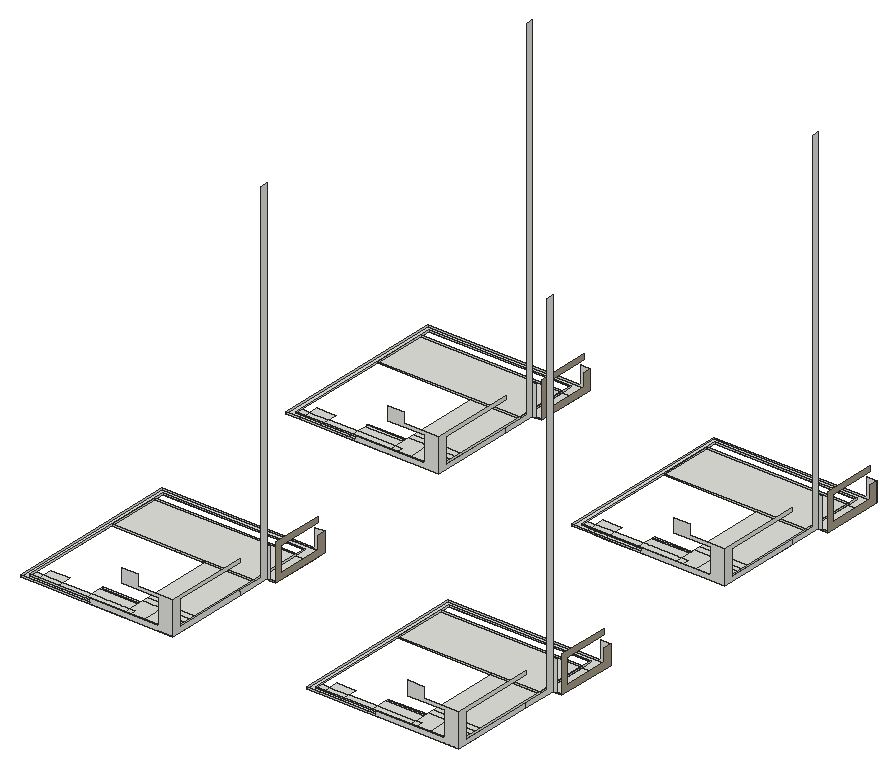
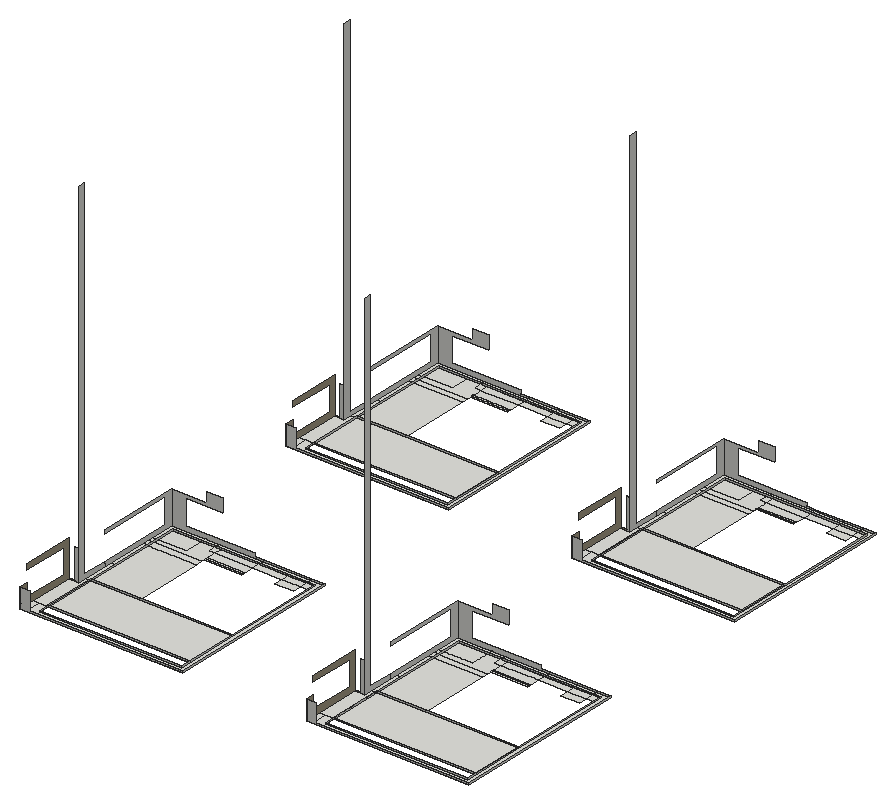
# SketchUp Ruby script. Lengths in inches.
U = 1.inch
M = Sketchup.active_model
def pt(a) = Geom::Point3d.new(a.map { |v| v * U })
def face(e, loops, mat)
  f = e.add_face(loops[0].map { |a| pt(a) })
  loops[1..].each { |l| e.add_face(l.map { |a| pt(a) }).erase! }
  f.material = f.back_material = mat if mat
  f
end
# faces: each face lists its corners as indices into pts; further lists are holes
def faces(e, pts, list, mat = nil) = list.each { |f| face(e, (f[0].is_a?(Array) ? f : [f]).map { |l| l.map { |i| pts[i] } }, mat) }
# xy, xz, yz: faces in a plane at the given z, y or x. An outline is a flat list of corners, or four numbers for a rectangle; further outlines are holes
def ring(l) = l.size == 4 ? [[l[0], l[1]], [l[2], l[1]], [l[2], l[3]], [l[0], l[3]]] : l.each_slice(2).to_a
def flat(e, list, mat, &to3) = list.each { |f| face(e, (f[0].is_a?(Array) ? f : [f]).map { |l| ring(l).map { |u, v| to3.(u, v) } }, mat) }
def xy(e, z, list, mat = nil) = flat(e, list, mat) { |x, y| [x, y, z] }
def xz(e, y, list, mat = nil) = flat(e, list, mat) { |x, z| [x, y, z] }
def yz(e, x, list, mat = nil) = flat(e, list, mat) { |y, z| [x, y, z] }
def lines(e, pts, list) = list.each { |a, b| e.add_line(pt(pts[a]), pt(pts[b])) }
# prism: a flat outline (further loops are holes) pulled along v
def prism(e, loops, v, mat = nil)
  f = face(e, loops, mat); d = Geom::Vector3d.new(v.map { |x| x * U })
  f.pushpull(f.normal.samedirection?(d) ? d.length : -d.length)
end
def box(e, o, s, mat = nil) = prism(e, [[o, [o[0] + s[0], o[1], o[2]], [o[0] + s[0], o[1] + s[1], o[2]], [o[0], o[1] + s[1], o[2]]]], [0, 0, s[2]], mat)
def at(x, y, z, deg = 0) = Geom::Transformation.translation(pt([x, y, z])) * Geom::Transformation.rotation(ORIGIN, Z_AXIS, deg.degrees)
def axes(o, x, y, z) = Geom::Transformation.new([*x, 0, *y, 0, *z, 0, *pt(o).to_a, 1])
def part(name) = M.definitions.add(name)
# library, detail: a bought-in or finely detailed component or shape, given as its bounding box
def library(name, o, s) = part(name).tap { |d| box(d.entities, o, s) }
def detail(e, o, s) = box(e.add_group.entities, o, s)
def put(e, d, t, mat = nil) = e.add_instance(d, t).tap { |i| i.material = mat if mat }
def group(e, t, mat = nil) = e.add_group.tap { |g| g.transformation = t; g.material = mat if mat }.entities
root = M.entities
M.materials.add("[Concrete Tile]").color = [165, 155, 133]
xy(root,252,[[262.875,1799.9375,262.875,2554.375,927.75,2554.375,927.75,2483.21,890.875,2483.21,890.875,2531.375,285.875,2531.375,285.875,1822.9375,319.53,1822.9375,319.53,1799.9375],[319.53,1799.9375,399.88,1822.9375],[399.88,1799.9375,523.04,1822.9375],[523.04,1799.9375,709.87,1822.9375],[709.87,1799.9375,767.19,1822.9375],
  [767.19,1799.9375,767.19,1822.9375,890.875,1822.9375,890.875,1902.66,913.875,1902.66,913.875,1799.9375],[1481.0625,1799.9375,1481.0625,2554.375,2145.9375,2554.375,2145.9375,2483.21,2109.0625,2483.21,2109.0625,2531.375,1504.0625,2531.375,1504.0625,1822.9375,1537.72,1822.9375,1537.72,1799.9375],[1537.72,1799.9375,1618.07,1822.9375],[1618.07,1799.9375,1741.23,1822.9375],[1741.23,1799.9375,1928.05,1822.9375],
  [1928.05,1799.9375,1985.38,1822.9375],[1985.38,1799.9375,1985.38,1822.9375,2109.0625,1822.9375,2109.0625,1902.66,2132.0625,1902.66,2132.0625,1799.9375],[285.875,1822.9375,319.53,1855.75],[319.53,1822.9375,399.88,1855.75],[399.88,1822.9375,523.04,1855.75],
  [523.04,1822.9375,683.6875,1855.75],[683.6875,1822.9375,709.87,1855.75],[709.87,1822.9375,767.19,1822.9375,767.19,1902.66,890.875,1902.66,890.875,1926.07,683.6875,1926.07,683.6875,1855.75,709.87,1855.75],[767.19,1822.9375,890.875,1902.66],[1504.0625,1822.9375,1537.72,1855.75],
  [1537.72,1822.9375,1618.07,1855.75],[1618.07,1822.9375,1741.23,1855.75],[1741.23,1822.9375,1901.875,1855.75],[1901.875,1822.9375,1928.05,1855.75],[1928.05,1822.9375,1985.38,1822.9375,1985.38,1902.66,2109.0625,1902.66,2109.0625,1926.07,1901.875,1926.07,1901.875,1855.75,1928.05,1855.75],
  [1985.38,1822.9375,2109.0625,1902.66],[319.53,1855.75,399.88,1893.25],[523.04,1855.75,683.6875,1897.5625],[1537.72,1855.75,1618.07,1893.25],[1741.23,1855.75,1901.875,1897.5625],
  [523.04,1897.5625,683.6875,1906.6875],[1741.23,1897.5625,1901.875,1906.6875],[890.875,1902.66,894.3125,1926.07],[894.3125,1902.66,913.875,1926.07],[2109.0625,1902.66,2112.5,1926.07],
  [2112.5,1902.66,2132.0625,1926.07],[523.04,1906.6875,683.6875,1913.4375],[1741.23,1906.6875,1901.875,1913.4375],[683.6875,1926.07,890.875,1953.7],[890.875,1926.07,894.3125,1953.7],
  [894.3125,1926.07,913.875,1953.7],[1901.875,1926.07,2109.0625,1953.7],[2109.0625,1926.07,2112.5,1953.7],[2112.5,1926.07,2132.0625,1953.7],[683.6875,1953.7,890.875,2258.18],
  [890.875,1953.7,890.875,2258.18,913.875,2258.18,913.875,2124.51,894.3125,2124.51,894.3125,1953.7],[894.3125,1953.7,913.875,2124.51],[1901.875,1953.7,2109.0625,2258.18],[2109.0625,1953.7,2109.0625,2258.18,2132.0625,2258.18,2132.0625,2124.51,2112.5,2124.51,2112.5,1953.7],[2112.5,1953.7,2132.0625,2124.51],
  [285.875,2258.18,890.875,2486.82],[890.875,2258.18,890.875,2483.21,954.6875,2483.21,954.6875,2295.875,913.875,2295.875,913.875,2258.18],[1504.0625,2258.18,2109.0625,2486.82],[2109.0625,2258.18,2109.0625,2483.21,2172.875,2483.21,2172.875,2295.875,2132.0625,2295.875,2132.0625,2258.18],[927.75,2483.21,954.6875,2554.375],
  [2145.9375,2483.21,2172.875,2554.375],[262.875,3214.625,262.875,3969.0625,927.75,3969.0625,927.75,3897.9,890.875,3897.9,890.875,3946.0625,285.875,3946.0625,285.875,3237.625,319.53,3237.625,319.53,3214.625],[319.53,3214.625,399.88,3237.625],[399.88,3214.625,523.04,3237.625],[523.04,3214.625,709.87,3237.625],
  [709.87,3214.625,767.19,3237.625],[767.19,3214.625,767.19,3237.625,890.875,3237.625,890.875,3317.34,913.875,3317.34,913.875,3214.625],[1481.0625,3214.625,1481.0625,3969.0625,2145.9375,3969.0625,2145.9375,3897.9,2109.0625,3897.9,2109.0625,3946.0625,1504.0625,3946.0625,1504.0625,3237.625,1537.72,3237.625,1537.72,3214.625],[1537.72,3214.625,1618.07,3237.625],[1618.07,3214.625,1741.23,3237.625],
  [1741.23,3214.625,1928.05,3237.625],[1928.05,3214.625,1985.38,3237.625],[1985.38,3214.625,1985.38,3237.625,2109.0625,3237.625,2109.0625,3317.34,2132.0625,3317.34,2132.0625,3214.625],[285.875,3237.625,319.53,3270.4375],[319.53,3237.625,399.88,3270.4375],
  [399.88,3237.625,523.04,3270.4375],[523.04,3237.625,683.6875,3270.4375],[683.6875,3237.625,709.87,3270.4375],[709.87,3237.625,767.19,3237.625,767.19,3317.34,890.875,3317.34,890.875,3340.76,683.6875,3340.76,683.6875,3270.4375,709.87,3270.4375],[767.19,3237.625,890.875,3317.34],
  [1504.0625,3237.625,1537.72,3270.4375],[1537.72,3237.625,1618.07,3270.4375],[1618.07,3237.625,1741.23,3270.4375],[1741.23,3237.625,1901.875,3270.4375],[1901.875,3237.625,1928.05,3270.4375],
  [1928.05,3237.625,1985.38,3237.625,1985.38,3317.34,2109.0625,3317.34,2109.0625,3340.76,1901.875,3340.76,1901.875,3270.4375,1928.05,3270.4375],[1985.38,3237.625,2109.0625,3317.34],[319.53,3270.4375,399.88,3307.9375],[523.04,3270.4375,683.6875,3312.25],[1537.72,3270.4375,1618.07,3307.9375],
  [1741.23,3270.4375,1901.875,3312.25],[523.04,3312.25,683.6875,3321.375],[1741.23,3312.25,1901.875,3321.375],[890.875,3317.34,894.3125,3340.76],[894.3125,3317.34,913.875,3340.76],
  [2109.0625,3317.34,2112.5,3340.76],[2112.5,3317.34,2132.0625,3340.76],[523.04,3321.375,683.6875,3328.125],[1741.23,3321.375,1901.875,3328.125],[683.6875,3340.76,890.875,3368.39],
  [890.875,3340.76,894.3125,3368.39],[894.3125,3340.76,913.875,3368.39],[1901.875,3340.76,2109.0625,3368.39],[2109.0625,3340.76,2112.5,3368.39],[2112.5,3340.76,2132.0625,3368.39],
  [683.6875,3368.39,890.875,3672.87],[890.875,3368.39,890.875,3672.87,913.875,3672.87,913.875,3539.2,894.3125,3539.2,894.3125,3368.39],[894.3125,3368.39,913.875,3539.2],[1901.875,3368.39,2109.0625,3672.87],[2109.0625,3368.39,2109.0625,3672.87,2132.0625,3672.87,2132.0625,3539.2,2112.5,3539.2,2112.5,3368.39],
  [2112.5,3368.39,2132.0625,3539.2],[285.875,3672.87,890.875,3901.51],[890.875,3672.87,890.875,3897.9,954.6875,3897.9,954.6875,3710.5625,913.875,3710.5625,913.875,3672.87],[1504.0625,3672.87,2109.0625,3901.51],[2109.0625,3672.87,2109.0625,3897.9,2172.875,3897.9,2172.875,3710.5625,2132.0625,3710.5625,2132.0625,3672.87],
  [927.75,3897.9,954.6875,3969.0625],[2145.9375,3897.9,2172.875,3969.0625]])
xz(root,1799.9375,[[262.875,252,319.53,258],[319.53,252,523.04,258],[523.04,252,557.4,258],[557.4,252,913.875,252,913.875,391.25,762.28,391.25,762.28,435.5,695.43,435.5,695.43,378,852.75,378,852.75,272.125,557.88,272.125,557.88,258,557.4,258],[1481.0625,252,1537.72,258],
  [1537.72,252,1741.23,258],[1741.23,252,1775.59,258],[1775.59,252,2132.0625,252,2132.0625,391.25,1980.47,391.25,1980.47,435.5,1913.62,435.5,1913.62,378,2070.9375,378,2070.9375,272.125,1776.07,272.125,1776.07,258,1775.59,258]])
xz(root,1822.9375,[[285.875,252,890.875,258],[1504.0625,252,2109.0625,258]])
xz(root,2258.18,[[285.875,252,683.6875,257.875],[683.6875,252,890.875,257.875],[1504.0625,252,1901.875,257.875],[1901.875,252,2109.0625,257.875]])
xz(root,2295.875,[[913.875,252,930.75,384],[2132.0625,252,2148.9375,384]])
xz(root,2295.875,[[930.75,252,954.6875,258],[2148.9375,252,2172.875,258]],"[Concrete Tile]")
xz(root,2486.82,[[285.875,252,890.875,257.875],[1504.0625,252,2109.0625,257.875]])
xz(root,2531.375,[[285.875,252,890.875,258],[1504.0625,252,2109.0625,258]])
xz(root,2554.375,[[262.875,252,262.875,258,913.875,258,913.875,336.0625,954.6875,336.0625,954.6875,252],[1481.0625,252,1481.0625,258,2132.0625,258,2132.0625,336.0625,2172.875,336.0625,2172.875,252]])
xz(root,3214.625,[[262.875,252,319.53,258],[319.53,252,523.04,258],[523.04,252,557.4,258],[557.4,252,913.875,252,913.875,391.25,762.28,391.25,762.28,435.5,695.43,435.5,695.43,378,852.75,378,852.75,272.125,557.88,272.125,557.88,258,557.4,258],[1481.0625,252,1537.72,258],
  [1537.72,252,1741.23,258],[1741.23,252,1775.59,258],[1775.59,252,2132.0625,252,2132.0625,391.25,1980.47,391.25,1980.47,435.5,1913.62,435.5,1913.62,378,2070.9375,378,2070.9375,272.125,1776.07,272.125,1776.07,258,1775.59,258]])
xz(root,3237.625,[[285.875,252,890.875,258],[1504.0625,252,2109.0625,258]])
xz(root,3672.87,[[285.875,252,683.6875,257.875],[683.6875,252,890.875,257.875],[1504.0625,252,1901.875,257.875],[1901.875,252,2109.0625,257.875]])
xz(root,3710.5625,[[913.875,252,930.75,384],[2132.0625,252,2148.9375,384]])
xz(root,3710.5625,[[930.75,252,954.6875,258],[2148.9375,252,2172.875,258]],"[Concrete Tile]")
xz(root,3901.51,[[285.875,252,890.875,257.875],[1504.0625,252,2109.0625,257.875]])
xz(root,3946.0625,[[285.875,252,890.875,258],[1504.0625,252,2109.0625,258]])
xz(root,3969.0625,[[262.875,252,262.875,258,913.875,258,913.875,336.0625,954.6875,336.0625,954.6875,252],[1481.0625,252,1481.0625,258,2132.0625,258,2132.0625,336.0625,2172.875,336.0625,2172.875,252]])
yz(root,262.875,[[1799.9375,252,2554.375,258],[3214.625,252,3969.0625,258]])
yz(root,285.875,[[1822.9375,252,2258.18,252,2258.18,257.875,2486.82,257.875,2486.82,252,2531.375,252,2531.375,258,1822.9375,258],[2258.18,252,2486.82,257.875],[3237.625,252,3672.87,252,3672.87,257.875,3901.51,257.875,3901.51,252,3946.0625,252,3946.0625,258,3237.625,258],[3672.87,252,3901.51,257.875]])
yz(root,890.875,[[1822.9375,252,1822.9375,258,2531.375,258,2531.375,252,2486.82,252,2486.82,257.875,2258.18,257.875,2258.18,252],[2258.18,252,2483.21,257.875],[2483.21,252,2486.82,257.875],[3237.625,252,3237.625,258,3946.0625,258,3946.0625,252,3901.51,252,3901.51,257.875,3672.87,257.875,3672.87,252],[3672.87,252,3897.9,257.875],
  [3897.9,252,3901.51,257.875]])
yz(root,913.875,[[1799.9375,252,2156.01,252,2156.01,271.5,1835.1875,271.5,1835.1875,378,2156.01,378,2156.01,391.25,1799.9375,391.25],[2156.01,252,2156.01,271.5,2266.33,271.5,2266.33,1764,2295.875,1764,2295.875,252],[3214.625,252,3570.7,252,3570.7,271.5,3249.875,271.5,3249.875,378,3570.7,378,3570.7,391.25,3214.625,391.25],[3570.7,252,3570.7,271.5,3681.01,271.5,3681.01,1764,3710.5625,1764,3710.5625,252]])
yz(root,954.6875,[[2295.875,252,2554.375,252,2554.375,336.0625,2518.89,336.0625,2518.89,280.3125,2321.98,280.3125,2321.98,384,2518.89,384,2518.89,408.0625,2295.875,408.0625],[3710.5625,252,3969.0625,252,3969.0625,336.0625,3933.57,336.0625,3933.57,280.3125,3736.67,280.3125,3736.67,384,3933.57,384,3933.57,408.0625,3710.5625,408.0625]],"[Concrete Tile]")
yz(root,1481.0625,[[1799.9375,252,2554.375,258],[3214.625,252,3969.0625,258]])
yz(root,1504.0625,[[1822.9375,252,2258.18,252,2258.18,257.875,2486.82,257.875,2486.82,252,2531.375,252,2531.375,258,1822.9375,258],[2258.18,252,2486.82,257.875],[3237.625,252,3672.87,252,3672.87,257.875,3901.51,257.875,3901.51,252,3946.0625,252,3946.0625,258,3237.625,258],[3672.87,252,3901.51,257.875]])
yz(root,2109.0625,[[1822.9375,252,1822.9375,258,2531.375,258,2531.375,252,2486.82,252,2486.82,257.875,2258.18,257.875,2258.18,252],[2258.18,252,2483.21,257.875],[2483.21,252,2486.82,257.875],[3237.625,252,3237.625,258,3946.0625,258,3946.0625,252,3901.51,252,3901.51,257.875,3672.87,257.875,3672.87,252],[3672.87,252,3897.9,257.875],
  [3897.9,252,3901.51,257.875]])
yz(root,2132.0625,[[1799.9375,252,2156.01,252,2156.01,271.5,1835.1875,271.5,1835.1875,378,2156.01,378,2156.01,391.25,1799.9375,391.25],[2156.01,252,2156.01,271.5,2266.33,271.5,2266.33,1764,2295.875,1764,2295.875,252],[3214.625,252,3570.7,252,3570.7,271.5,3249.875,271.5,3249.875,378,3570.7,378,3570.7,391.25,3214.625,391.25],[3570.7,252,3570.7,271.5,3681.01,271.5,3681.01,1764,3710.5625,1764,3710.5625,252]])
yz(root,2172.875,[[2295.875,252,2554.375,252,2554.375,336.0625,2518.89,336.0625,2518.89,280.3125,2321.98,280.3125,2321.98,384,2518.89,384,2518.89,408.0625,2295.875,408.0625],[3710.5625,252,3969.0625,252,3969.0625,336.0625,3933.57,336.0625,3933.57,280.3125,3736.67,280.3125,3736.67,384,3933.57,384,3933.57,408.0625,3710.5625,408.0625]],"[Concrete Tile]")
p = [[2112.5,1835.1875,271.5],[2112.5,1835.1875,252],[894.3125,1835.1875,271.5],[894.3125,1835.1875,252],[2112.5,3249.875,271.5],[2112.5,3249.875,252],
  [894.3125,3249.875,271.5],[894.3125,3249.875,252]]
lines(root,p,[[0,1],[2,3],[4,5],[6,7]])
